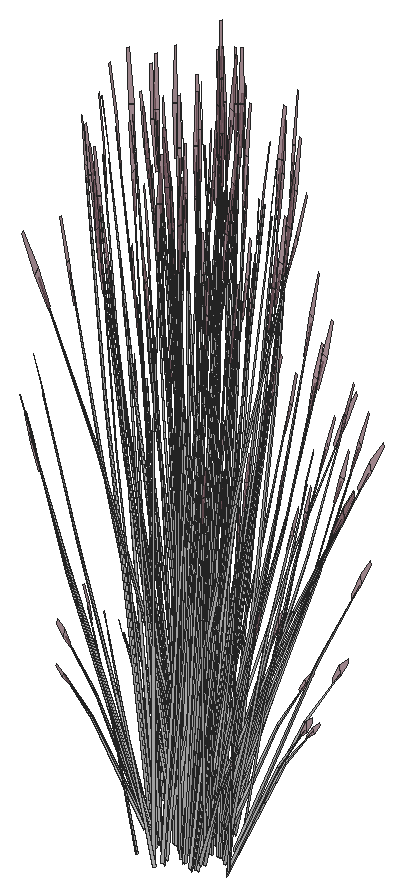
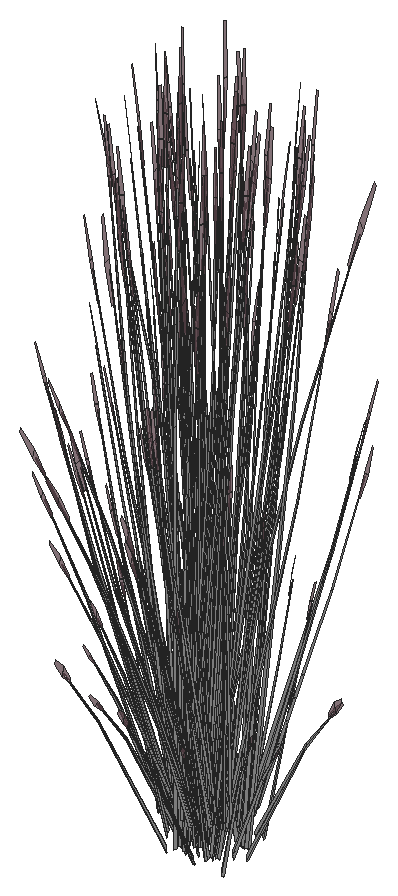
# SketchUp Ruby script. Lengths in inches.
U = 1.inch
M = Sketchup.active_model
def pt(a) = Geom::Point3d.new(a.map { |v| v * U })
def face(e, loops, mat)
  f = e.add_face(loops[0].map { |a| pt(a) })
  loops[1..].each { |l| e.add_face(l.map { |a| pt(a) }).erase! }
  f.material = f.back_material = mat if mat
  f
end
# faces: each face lists its corners as indices into pts; further lists are holes
def faces(e, pts, list, mat = nil) = list.each { |f| face(e, (f[0].is_a?(Array) ? f : [f]).map { |l| l.map { |i| pts[i] } }, mat) }
# xy, xz, yz: faces in a plane at the given z, y or x. An outline is a flat list of corners, or four numbers for a rectangle; further outlines are holes
def ring(l) = l.size == 4 ? [[l[0], l[1]], [l[2], l[1]], [l[2], l[3]], [l[0], l[3]]] : l.each_slice(2).to_a
def flat(e, list, mat, &to3) = list.each { |f| face(e, (f[0].is_a?(Array) ? f : [f]).map { |l| ring(l).map { |u, v| to3.(u, v) } }, mat) }
def xy(e, z, list, mat = nil) = flat(e, list, mat) { |x, y| [x, y, z] }
def xz(e, y, list, mat = nil) = flat(e, list, mat) { |x, z| [x, y, z] }
def yz(e, x, list, mat = nil) = flat(e, list, mat) { |y, z| [x, y, z] }
def lines(e, pts, list) = list.each { |a, b| e.add_line(pt(pts[a]), pt(pts[b])) }
# prism: a flat outline (further loops are holes) pulled along v
def prism(e, loops, v, mat = nil)
  f = face(e, loops, mat); d = Geom::Vector3d.new(v.map { |x| x * U })
  f.pushpull(f.normal.samedirection?(d) ? d.length : -d.length)
end
def box(e, o, s, mat = nil) = prism(e, [[o, [o[0] + s[0], o[1], o[2]], [o[0] + s[0], o[1] + s[1], o[2]], [o[0], o[1] + s[1], o[2]]]], [0, 0, s[2]], mat)
def at(x, y, z, deg = 0) = Geom::Transformation.translation(pt([x, y, z])) * Geom::Transformation.rotation(ORIGIN, Z_AXIS, deg.degrees)
def axes(o, x, y, z) = Geom::Transformation.new([*x, 0, *y, 0, *z, 0, *pt(o).to_a, 1])
def part(name) = M.definitions.add(name)
# library, detail: a bought-in or finely detailed component or shape, given as its bounding box
def library(name, o, s) = part(name).tap { |d| box(d.entities, o, s) }
def detail(e, o, s) = box(e.add_group.entities, o, s)
def put(e, d, t, mat = nil) = e.add_instance(d, t).tap { |i| i.material = mat if mat }
def group(e, t, mat = nil) = e.add_group.tap { |g| g.transformation = t; g.material = mat if mat }.entities
root = M.entities
M.materials.add("LightPink_Translucent").color = [144, 107, 117]
M.materials["LightPink_Translucent"].alpha = 0.75
M.materials.add("[_0053_Ivory_]").color = [200, 200, 200]
c1 = part("blade")
p = [[2.15,0.21,22],[0,0.17,0],[0.09,0.45,0],[2.18,0.31,22],[2.29,0.31,22],[0.38,0.45,0],
  [2.48,0.24,33],[2.49,0.24,33],[2.48,0.22,33]]
faces(c1.entities,p,[[0,1,2,3],[4,5,2,3],[6,3,4,7],[8,0,3,6]])
c2 = part("seeds")
p = [[0.3,-0.1,1.38],[-0.01,-0.03,1.59],[-0.01,-0.03,0.03],[0.14,-0.07,-0.07],[0.29,-0.03,3],[0.15,0.01,3.11]]
faces(c2.entities,p,[[0,1,2,3],[1,0,4,5]],"LightPink_Translucent")
c3 = part("blade with seeds")
put(c3.entities,c1,at(0,0,0))
put(c3.entities,c2,axes([2.4,0.25,30.99],[1.5799,-0.05474,1.17369],[-0.12525,1.92788,0.29478],[-0.07173,-0.02425,1.56792]))
put(root,c3,axes([642.65,204.3,131.33],[-0.59932,0.14948,-0.51099],[-0.10484,-0.56611,-0.3958],[-0.16097,-0.16223,0.97773]),"[_0053_Ivory_]")
put(root,c3,axes([646.1875,205.65,131.63],[0.31725,-0.49618,-0.71045],[0.55593,0.35263,0.08574],[0.18942,-0.17977,1.00501]),"[_0053_Ivory_]")
put(root,c3,axes([642.76,204.21,129.03],[-0.37973,-0.63014,0],[0.6353,-0.35142,-0.51607],[0.14469,-0.08004,1.63711]),"[_0053_Ivory_]")
put(root,c3,axes([646.17,205.42,131.33],[-0.15602,-0.5742,-0.51099],[0.59087,-0.10045,-0.3958],[0.16933,-0.15423,0.97773]),"[_0053_Ivory_]")
put(root,c3,axes([643.59,203.45,128.78],[-0.4197,0.36076,-0.03893],[-0.38456,-0.39511,-0.17649],[-0.02707,-0.11196,0.58215]),"[_0053_Ivory_]")
put(root,c3,axes([644.13,207.72,129.98],[0.52485,0.25358,1.51261],[-0.51417,0.54629,0.59816],[-0.23031,-0.32378,1.26806]),"[_0053_Ivory_]")
put(root,c3,axes([641.39,205.97,128.67],[0,-0.62885,-0.49651],[0.67951,0,0],[0,-0.14322,1.57504]),"[_0053_Ivory_]")
put(root,c3,axes([643.27,204.11,128.67],[0.56842,-0.31443,-0.49651],[0.33976,0.56381,0],[0.12946,-0.07161,1.57504]),"[_0053_Ivory_]")
put(root,c3,axes([646.65,205.2,129.24],[-0.21697,-0.01863,1.43002],[-0.22228,-0.49966,-0.30754],[0.26655,-0.14135,0.61141]),"[_0053_Ivory_]")
put(root,c3,axes([643.95,205.4,128.71],[0.40909,-0.47266,-0.62353],[0.50819,0.4286,-0.16365],[0.16393,-0.11791,1.37633]),"[_0053_Ivory_]")
put(root,c3,axes([646.9,204.28,129.42],[-0.2023,0.32011,1.1486],[-0.17388,-0.43009,0.84392],[0.16708,-0.10777,0.25299]),"[_0053_Ivory_]")
put(root,c3,axes([646.61,205.48,131.18],[0.52868,-0.08987,-0.35414],[0.1396,0.51376,0.4572],[0.1515,-0.13799,0.87481]),"[_0053_Ivory_]")
put(root,c3,axes([643.24,206.23,128.86],[0.29468,-0.56664,-0.44739],[0.61229,0.27271,0.21531],[0,-0.13062,1.43643]),"[_0053_Ivory_]")
put(root,c3,axes([641.47,204.77,131.18],[-0.34557,-0.39372,-0.35414],[0.39459,-0.37271,0.4572],[-0.20048,-0.05671,0.87481]),"[_0053_Ivory_]")
put(root,c3,axes([643.5,205.95,129.32],[-0.07077,-0.71755,-0.29095],[0.73712,-0.04339,-0.50002],[0.1298,-0.09558,1.59708]),"[_0053_Ivory_]")
put(root,c3,axes([641.68,205.98,128.68],[0.42396,-0.39235,-0.30978],[0.42396,0.39235,0.30978],[0,-0.12637,1.38974]),"[_0053_Ivory_]")
put(root,c3,axes([641.51,204.1,128.78],[-0.1752,0.51349,-0.03893],[-0.53924,-0.15795,-0.17649],[-0.08187,-0.08399,0.58215]),"[_0053_Ivory_]")
put(root,c3,axes([643.16,206.7,129.32],[-0.68399,-0.30005,-0.29095],[0.32934,-0.63331,-0.50002],[-0.0215,-0.15549,1.59708]),"[_0053_Ivory_]")
put(root,c3,axes([641.22,206.45,129.03],[-0.75945,0,0],[0,-0.70283,-0.51607],[0,-0.16007,1.63711]),"[_0053_Ivory_]")
put(root,c3,axes([643.41,204.36,128.68],[0.56663,0.1556,-0.30978],[-0.14267,0.54795,0.30978],[0.11423,-0.06319,1.38974]),"[_0053_Ivory_]")
put(root,c3,axes([641.8,206.26,128.98],[-0.56493,0.5287,0.30756],[-0.56528,-0.52313,-0.36492],[-0.01973,-0.15014,1.64885]),"[_0053_Ivory_]")
put(root,c3,axes([643.6,206.51,129.09],[0.68433,0.30479,0.24065],[-0.32934,0.63331,0.50002],[0,-0.14599,1.60543]),"[_0053_Ivory_]")
put(root,c3,axes([643.33,207.37,129.09],[0.16098,-0.74515,-0.23429],[0.76326,0.12989,0.51271],[-0.13337,-0.1029,1.5644]),"[_0053_Ivory_]")
put(root,c3,axes([641.63,205.17,131.33],[-0.44101,0.41656,-0.51099],[-0.38623,-0.44004,-0.3958],[-0.22407,-0.06338,0.97773]),"[_0053_Ivory_]")
put(root,c3,axes([640.64,205.72,129.42],[0.38775,-0.045,1.1486],[-0.24596,0.39648,0.84392],[-0.19161,-0.05948,0.25299]),"[_0053_Ivory_]")
put(root,c3,axes([643.38,206.08,129.37],[-0.65953,0.03882,0.44739],[-0.05964,-0.64439,-0.21531],[0.11807,-0.06531,1.43643]),"[_0053_Ivory_]")
put(root,c3,axes([641.68,206.55,129.13],[0,0.62885,0.49651],[-0.67951,0,0],[0,-0.14322,1.57504]),"[_0053_Ivory_]")
put(root,c3,axes([646.45,206.69,131.33],[0.16454,-0.57202,-0.51099],[0.56413,0.19607,-0.3958],[0.22713,-0.05245,0.97773]),"[_0053_Ivory_]")
put(root,c3,axes([645.55,204.37,129.03],[0.37973,-0.63014,0],[0.6353,0.35142,-0.51607],[0.14469,0.08004,1.63711]),"[_0053_Ivory_]")
put(root,c3,axes([643.28,207.0625,128.86],[-0.36485,-0.52782,-0.44739],[0.55265,-0.37168,0.21531],[-0.11807,-0.06531,1.43643]),"[_0053_Ivory_]")
put(root,c3,axes([643.36,206.32,129.01],[0.26406,0.70318,0.45755],[-0.7545,0.24452,0.17955],[0.00922,-0.12921,1.58856]),"[_0053_Ivory_]")
put(root,c3,axes([647.05,206.86,128.64],[-0.39118,0.07547,1.41583],[-0.06226,-0.6007,0.08104],[0.27398,-0.09092,0.80566]),"[_0053_Ivory_]")
put(root,c3,axes([647.76,206.32,128.91],[-0.37654,-0.40212,-0.06488],[0.4124,-0.36845,-0.29416],[0.11685,-0.02594,0.97024]),"[_0053_Ivory_]")
put(root,c3,axes([643.22,206.87,129.37],[-0.29468,0.56664,0.44739],[-0.61229,-0.27271,-0.21531],[0,-0.13062,1.43643]),"[_0053_Ivory_]")
put(root,c3,axes([644.31,206.375,128.86],[0,-0.72763,0],[0.75945,0,0],[0,0,1.79456]),"[_0053_Ivory_]")
put(root,c3,axes([645.23,204.69,129.13],[-0.56842,-0.31443,0.49651],[0.33976,-0.56381,0],[0.12946,0.07161,1.57504]),"[_0053_Ivory_]")
put(root,c3,axes([646.34,206.9,131.63],[0.53369,-0.27773,-0.71045],[0.29743,0.5717,0.08574],[0.25786,-0.06494,1.00501]),"[_0053_Ivory_]")
put(root,c3,axes([642.95,207.26,128.71],[-0.63179,-0.1031,-0.62353],[0.13332,-0.63596,-0.16365],[-0.18854,-0.07706,1.37633]),"[_0053_Ivory_]")
put(root,c3,axes([643.95,205.92,129.01],[-0.50358,0.57069,0.45755],[-0.59827,-0.50377,0.17955],[0.1214,-0.05695,1.58856]),"[_0053_Ivory_]")
put(root,c3,axes([644.5,206.94,128.95],[-0.56493,-0.54126,-0.06131],[0.56528,-0.54159,0],[-0.01973,-0.0189,1.75571]),"[_0053_Ivory_]")
put(root,c3,axes([643.07,204.98,129.13],[-0.17545,0.62497,0.17642],[-0.64204,-0.17686,0.35086],[0.11091,-0.00304,1.60407]),"[_0053_Ivory_]")
put(root,c3,axes([642.81,205.48,128.25],[-0.59782,0.25177,1.28929],[-0.19028,-0.72239,0.50096],[0.36709,0.01202,1.46642]),"[_0053_Ivory_]")
put(root,c3,axes([644.41,205.67,129.27],[0.11717,-0.56122,0.1448],[0.57245,0.09742,-0.41347],[0.10418,0.05763,1.26744]),"[_0053_Ivory_]")
put(root,c3,axes([643.42,207.01,129.01],[0.76764,0.13249,0.45755],[-0.15622,0.74829,0.17955],[-0.11218,-0.07226,1.58856]),"[_0053_Ivory_]")
put(root,c3,axes([647.48,206.46,128.15],[-0.03174,-0.09547,1.76342],[0.22015,-0.55846,-0.26939],[0.22208,-0.00803,0.30037]),"[_0053_Ivory_]")
put(root,c3,axes([640.92,206.37,128.15],[0.0154,0.09911,1.76342],[-0.31051,0.51756,-0.26939],[-0.22056,-0.02609,0.30037]),"[_0053_Ivory_]")
put(root,c3,axes([644.17,205.82,129.37],[-0.36485,-0.52782,0.44739],[0.55265,-0.37168,-0.21531],[0.11807,0.06531,1.43643]),"[_0053_Ivory_]")
put(root,c3,axes([642.28,208.23,128.68],[-0.14267,-0.54795,-0.30978],[0.56663,-0.1556,0.30978],[-0.11423,-0.06319,1.38974]),"[_0053_Ivory_]")
put(root,c3,axes([643.01,208.2,129.13],[0.65264,-0.16691,0.17642],[0.16115,0.62115,0.35086],[-0.05821,-0.0905,1.60407]),"[_0053_Ivory_]")
put(root,c3,axes([644.35,205.86,129.32],[0.61322,-0.4175,-0.29095],[0.40778,0.58992,-0.50002],[0.1513,0.05991,1.59708]),"[_0053_Ivory_]")
put(root,c3,axes([646.79,206.96,131.18],[0.50475,0.17543,-0.35414],[-0.14722,0.5118,0.4572],[0.20322,-0.04693,0.87481]),"[_0053_Ivory_]")
put(root,c3,axes([642.125,208.47,128.67],[-0.56842,-0.31443,-0.49651],[0.33976,-0.56381,0],[-0.12946,-0.07161,1.57504]),"[_0053_Ivory_]")
put(root,c3,axes([645.9,204.75,128.67],[0.56842,0.31443,-0.49651],[-0.33976,0.56381,0],[0.12946,0.07161,1.57504]),"[_0053_Ivory_]")
put(root,c3,axes([644.82,206.54,128.86],[0.67951,0,0],[0,0.65103,0],[0,0,1.78407]),"[_0053_Ivory_]")
put(root,c3,axes([643.67,207.36,129.32],[-0.61322,0.4175,-0.29095],[-0.40778,-0.58992,-0.50002],[-0.1513,-0.05991,1.59708]),"[_0053_Ivory_]")
put(root,c3,axes([645.01,205.01,129.13],[-0.65264,0.16691,0.17642],[-0.16115,-0.62115,0.35086],[0.05821,0.0905,1.60407]),"[_0053_Ivory_]")
put(root,c3,axes([645.42,206.32,130.53],[-0.25192,0.01424,1.71376],[0.16712,-0.61729,0.13857],[0.35901,0.03818,0.73262]),"[_0053_Ivory_]")
put(root,c3,axes([645.74,204.98,128.68],[0.14267,0.54795,-0.30978],[-0.56663,0.1556,0.30978],[0.11423,0.06319,1.38974]),"[_0053_Ivory_]")
put(root,c3,axes([644.6,206.21,129.03],[-0.76764,-0.13249,0.49198],[0.15622,-0.74829,0.19306],[0.11218,0.07226,1.70813]),"[_0053_Ivory_]")
put(root,c3,axes([643.99,208.05,128.86],[-0.19817,-0.54216,0],[0.56587,-0.18986,0],[0,0,1.54371]),"[_0053_Ivory_]")
put(root,c3,axes([643.61,207.54,129.27],[-0.11717,0.56122,0.1448],[-0.57245,-0.09742,-0.41347],[-0.10418,-0.05763,1.26744]),"[_0053_Ivory_]")
put(root,c3,axes([644.73,207.98,128.84],[0.63764,-0.21337,-0.19198],[0.22406,0.61462,0.00008],[0.07038,-0.02358,1.73897]),"[_0053_Ivory_]")
put(root,c3,axes([644.95,208.24,129.13],[0.17545,-0.62497,0.17642],[0.64204,0.17686,0.35086],[-0.11091,0.00304,1.60407]),"[_0053_Ivory_]")
put(root,c3,axes([644.81,206.82,128.87],[0.42396,0.40619,0],[-0.42396,0.40619,0],[0,0,1.69266]),"[_0053_Ivory_]")
put(root,c3,axes([645.95,206.64,129.13],[-0.47719,-0.45806,0.17642],[0.48088,-0.44429,0.35086],[-0.0527,0.09355,1.60407]),"[_0053_Ivory_]")
put(root,c3,axes([645.07,205.95,128.71],[0.63179,0.1031,-0.62353],[-0.13332,0.63596,-0.16365],[0.18854,0.07706,1.37633]),"[_0053_Ivory_]")
put(root,c3,axes([647.86,207.06,129.42],[-0.37526,0.10382,1.1486],[0.17664,-0.42906,0.84392],[0.19907,0.02936,0.25299]),"[_0053_Ivory_]")
put(root,c3,axes([643.85,208.3,128.85],[-0.61229,-0.28233,0],[0.29468,-0.58663,0],[0,0,1.62707]),"[_0053_Ivory_]")
put(root,c3,axes([644.36,207.55,129.12],[-0.59306,-0.50614,-0.25192],[0.49904,-0.56836,0.5513],[-0.1597,0.05921,1.68216]),"[_0053_Ivory_]")
put(root,c3,axes([642.8,208.52,129.13],[0.56842,0.31443,0.49651],[-0.33976,0.56381,0],[-0.12946,-0.07161,1.57504]),"[_0053_Ivory_]")
put(root,c3,axes([644.8,206.34,129.37],[0.29468,-0.56664,0.44739],[0.61229,0.27271,-0.21531],[0,0.13062,1.43643]),"[_0053_Ivory_]")
put(root,c3,axes([644.6875,206.67,128.95],[0,0.72727,-0.05637],[-0.75945,0,0],[0,0.02286,1.79368]),"[_0053_Ivory_]")
put(root,c3,axes([644.74,206.15,128.86],[0.36485,0.52782,-0.44739],[-0.55265,0.37168,0.21531],[0.11807,0.06531,1.43643]),"[_0053_Ivory_]")
put(root,c3,axes([647.21,208.38,130.58],[-0.11624,-0.52862,-0.03492],[0.54943,-0.12153,-0.15832],[0.11473,0.03351,0.52218]),"[_0053_Ivory_]")
put(root,c3,axes([642.47,208.85,129.03],[-0.37973,0.63014,0],[-0.6353,-0.35142,-0.51607],[-0.14469,-0.08004,1.63711]),"[_0053_Ivory_]")
put(root,c3,axes([646.35,206.66,129.13],[0,-0.62885,0.49651],[0.67951,0,0],[0,0.14322,1.57504]),"[_0053_Ivory_]")
put(root,c3,axes([644.65,207.13,129.37],[0.65953,-0.03882,0.44739],[0.05964,0.64439,-0.21531],[-0.11807,0.06531,1.43643]),"[_0053_Ivory_]")
put(root,c3,axes([645.06,206.47,129.27],[0.56587,-0.18339,0.1448],[0.19817,0.52368,-0.41347],[0,0.11525,1.26744]),"[_0053_Ivory_]")
put(root,c3,axes([644.06,207.44,128.86],[-0.65953,0.03882,-0.44739],[-0.05964,-0.64439,0.21531],[-0.11807,0.06531,1.43643]),"[_0053_Ivory_]")
put(root,c3,axes([647.16,207.75,129.24],[-0.14627,-0.15466,1.43002],[0.19032,-0.51164,-0.30754],[0.29594,0.06931,0.61141]),"[_0053_Ivory_]")
put(root,c3,axes([644.55,208.3125,128.86],[0.61229,0.28233,0],[-0.29468,0.58663,0],[0,0,1.74954]),"[_0053_Ivory_]")
put(root,c3,axes([644.79,208.94,128.85],[-0.37499,-0.63235,-0.05142],[0.6353,-0.35142,0.51607],[-0.15655,0.0602,1.6363]),"[_0053_Ivory_]")
put(root,c3,axes([644.66,207.41,129.27],[0.44871,0.37783,0.1448],[-0.37428,0.42627,-0.41347],[-0.10418,0.05763,1.26744]),"[_0053_Ivory_]")
put(root,c3,axes([645.82,208.06,131.63],[0.60713,0.01514,-0.71045],[-0.04078,0.63759,0.08574],[0.25721,0.06729,1.00501]),"[_0053_Ivory_]")
put(root,c3,axes([645.13,208.57,129.13],[0.56842,-0.31443,0.49651],[0.33976,0.56381,0],[-0.12946,0.07161,1.57504]),"[_0053_Ivory_]")
put(root,c3,axes([644.32,208.07,128.94],[0.26406,0.72244,-0.06012],[-0.7545,0.25315,0],[0.00922,0.02523,1.72173]),"[_0053_Ivory_]")
put(root,c3,axes([644.62,208.86,128.68],[-0.56663,-0.1556,-0.30978],[0.14267,-0.54795,0.30978],[-0.11423,0.06319,1.38974]),"[_0053_Ivory_]")
put(root,c3,axes([646.81,206.77,129.03],[0.75945,0,0],[0,0.70283,-0.51607],[0,0.16007,1.63711]),"[_0053_Ivory_]")
put(root,c3,axes([646.51,207.125,128.85],[-0.75908,-0.00503,-0.04976],[0,-0.70283,0.49943],[-0.02386,0.16,1.58352]),"[_0053_Ivory_]")
put(root,c3,axes([644.86,206.51,129.32],[0.68399,0.30005,-0.29095],[-0.32934,0.63331,-0.50002],[0.0215,0.15549,1.59708]),"[_0053_Ivory_]")
put(root,c3,axes([640.09,208.85,129.42],[0.25312,-0.28501,1.1486],[0.09988,0.45119,0.84392],[-0.18292,0.08079,0.25299]),"[_0053_Ivory_]")
put(root,c3,axes([646.18,208.32,131.18],[0.34557,0.39372,-0.35414],[-0.39459,0.37271,0.4572],[0.20048,0.05671,0.87481]),"[_0053_Ivory_]")
put(root,c3,axes([646.35,207.23,128.68],[-0.42396,0.39235,-0.30978],[-0.42396,-0.39235,0.30978],[0,0.12637,1.38974]),"[_0053_Ivory_]")
put(root,c3,axes([644.52,207.27,129.32],[0.07077,0.71755,-0.29095],[-0.73712,0.04339,-0.50002],[-0.1298,0.09558,1.59708]),"[_0053_Ivory_]")
put(root,c3,axes([644.79,206.99,128.86],[-0.29468,0.56664,-0.44739],[-0.61229,-0.27271,0.21531],[0,0.13062,1.43643]),"[_0053_Ivory_]")
put(root,c3,axes([641.04,207.62,131.18],[-0.52868,0.08987,-0.35414],[-0.1396,-0.51376,0.4572],[-0.1515,0.13799,0.87481]),"[_0053_Ivory_]")
put(root,c3,axes([644.08,207.8125,128.71],[-0.40909,0.47266,-0.62353],[-0.50819,-0.4286,-0.16365],[-0.16393,0.11791,1.37633]),"[_0053_Ivory_]")
put(root,c3,axes([644.81,208.61,128.98],[0.76036,0.2044,0.30756],[-0.19023,0.7306,-0.36492],[-0.12585,0.09144,1.64885]),"[_0053_Ivory_]")
put(root,c3,axes([644.75,209.1,128.67],[-0.56842,0.31443,-0.49651],[-0.33976,-0.56381,0],[-0.12946,0.07161,1.57504]),"[_0053_Ivory_]")
put(root,c3,axes([646.64,207.24,128.67],[0,0.62885,-0.49651],[-0.67951,0,0],[0,0.14322,1.57504]),"[_0053_Ivory_]")
put(root,c3,axes([644.94,207.3125,130.53],[-0.2256,-0.10835,1.71376],[0.46687,-0.45453,0.13857],[0.29098,0.20505,0.73262]),"[_0053_Ivory_]")
put(root,c3,axes([645.78,208.55,129.42],[-0.34197,-0.18082,1.1486],[0.44156,-0.18372,0.84392],[0.1191,0.15563,0.25299]),"[_0053_Ivory_]")
put(root,c3,axes([641.96,207.11,130.53],[0.1517,-0.19322,1.71376],[0.38303,0.52154,0.13857],[-0.26271,0.23751,0.73262]),"[_0053_Ivory_]")
put(root,c3,axes([641.48,207.68,131.33],[0.15602,0.5742,-0.51099],[-0.59087,0.10045,-0.3958],[-0.16933,0.15423,0.97773]),"[_0053_Ivory_]")
put(root,c3,axes([645.27,209.01,129.03],[0.37973,0.63014,0],[-0.6353,0.35142,-0.51607],[-0.14469,0.08004,1.63711]),"[_0053_Ivory_]")
put(root,c3,axes([645.87,209.22,128.15],[0.04425,-0.09079,1.76342],[0.55709,-0.26738,-0.26939],[0.16889,0.13839,0.30037]),"[_0053_Ivory_]")
put(root,c3,axes([644.94,206.51,129.5],[-0.01659,-0.59209,1.41272],[0.75089,0.15348,0.59816],[-0.1776,0.32398,1.3335]),"[_0053_Ivory_]")
put(root,c3,axes([645.14,207.16,128.75],[0.2227,0.57576,-0.69212],[-0.64151,0.20736,-0.18165],[0.02462,0.19497,1.52773]),"[_0053_Ivory_]")
put(root,c3,axes([640.76,209.14,128.15],[0.08147,0.06283,1.76342],[0.13814,0.58211,-0.26939],[-0.18056,0.12413,0.30037]),"[_0053_Ivory_]")
put(root,c3,axes([645,208.8,131.33],[0.59932,-0.14948,-0.51099],[0.10484,0.56611,-0.3958],[0.16097,0.16223,0.97773]),"[_0053_Ivory_]")
put(root,c3,axes([645.83,209.37,129.32],[-0.38947,-0.01972,1.0506],[0.25721,-0.41888,0.58006],[0.15386,0.14882,0.8241]),"[_0053_Ivory_]")
put(root,c3,axes([641.84,207.59,130.53],[0.11309,-0.21615,1.71376],[0.47441,0.44731,0.13857],[-0.21402,0.27879,0.73262]),"[_0053_Ivory_]")
put(root,c3,axes([644.56,208.35,129.24],[0.01072,-0.20846,1.43002],[0.51218,-0.23285,-0.30754],[0.15811,0.2495,0.61141]),"[_0053_Ivory_]")
put(root,c3,axes([641.97,208.81,131.18],[-0.41095,0.33109,-0.35414],[-0.38901,-0.37805,0.4572],[-0.05919,0.19208,0.87481]),"[_0053_Ivory_]")
put(root,c3,axes([642.24,210.09,129.42],[-0.01572,-0.37392,1.1486],[0.39276,0.26669,0.84392],[-0.07724,0.17822,0.25299]),"[_0053_Ivory_]")
put(root,c3,axes([643.27,209.2,128.15],[0.09829,-0.03422,1.76342],[0.59126,0.18834,-0.26939],[0.01729,0.21228,0.30037]),"[_0053_Ivory_]")
put(root,c3,axes([642.38,208.65,131.66],[0.43478,0.42253,-0.5672],[-0.45929,0.37004,-0.43934],[-0.06615,0.21468,1.08528]),"[_0053_Ivory_]")
put(root,c3,axes([641.91,209.28,129.48],[0.55175,-0.11136,0.06507],[0.12684,0.44864,-0.86304],[-0.03498,0.22711,0.7736]),"[_0053_Ivory_]")
put(root,c3,axes([643.67,209.06,131.33],[0.59704,0.15764,-0.51099],[-0.20464,0.54049,-0.3958],[0.05475,0.21761,0.97773]),"[_0053_Ivory_]")
put(root,c3,axes([644.01,207.94,130.53],[-0.13883,-0.2019,1.71376],[0.64153,-0.16998,0.13857],[0.14499,0.31697,0.73262]),"[_0053_Ivory_]")
put(root,c3,axes([643.4,209.39,131.18],[-0.1831,0.48359,-0.35414],[-0.53419,-0.14105,0.4572],[0.04898,0.1947,0.87481]),"[_0053_Ivory_]")
put(root,c3,axes([642.25,208.46,131.99],[-0.0158,0.58168,-0.7886],[-0.66548,-0.03907,0.09517],[-0.07023,0.24643,1.11556]),"[_0053_Ivory_]")
put(root,c3,axes([642.88,208.04,130.53],[-0.01487,-0.24136,1.71376],[0.64429,0.16012,0.13857],[-0.03985,0.34396,0.73262]),"[_0053_Ivory_]")
put(root,c3,axes([643.46,208.96,131.63],[0.28988,0.51132,-0.71045],[-0.59671,0.28496,0.08574],[0.06778,0.24706,1.00501]),"[_0053_Ivory_]")
put(root,c3,axes([641.78,209.76,129.24],[0.19166,-0.0992,1.43002],[0.4732,0.29912,-0.30754],[-0.14084,0.25882,0.61141]),"[_0053_Ivory_]")
put(root,c3,axes([642.03,209.28,130.02],[0.01334,-0.32463,1.54345],[0.60018,0.17147,0.21329],[-0.052,0.34598,0.72882]),"[_0053_Ivory_]")
